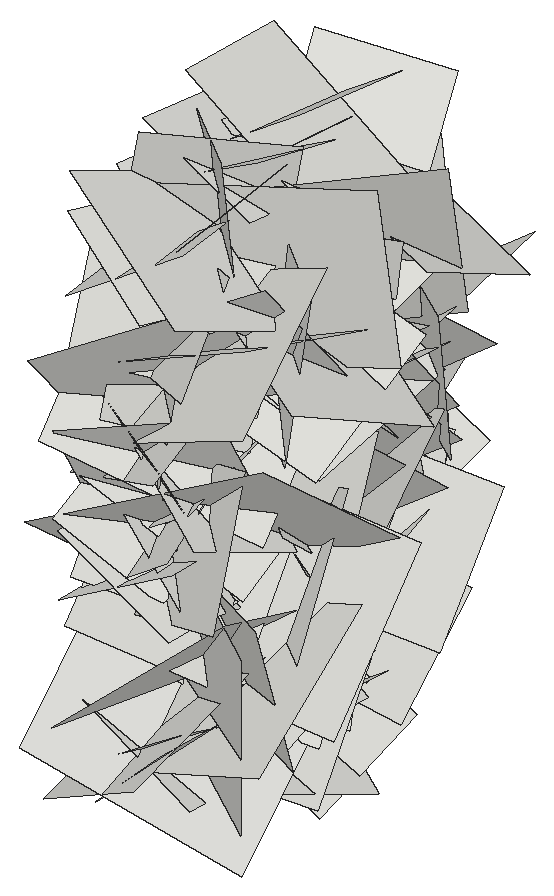
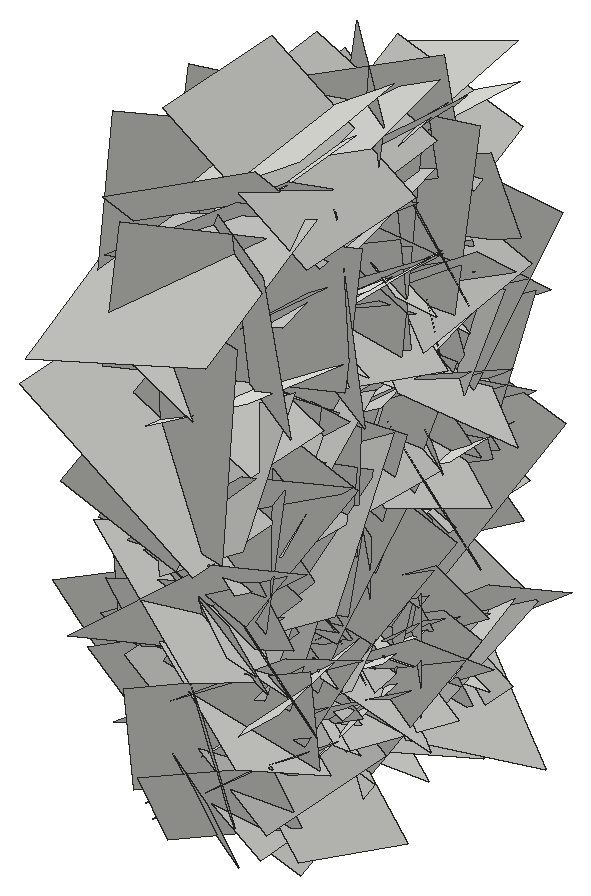
# SketchUp Ruby script. Lengths in inches.
U = 1.inch
M = Sketchup.active_model
def pt(a) = Geom::Point3d.new(a.map { |v| v * U })
def face(e, loops, mat)
  f = e.add_face(loops[0].map { |a| pt(a) })
  loops[1..].each { |l| e.add_face(l.map { |a| pt(a) }).erase! }
  f.material = f.back_material = mat if mat
  f
end
# faces: each face lists its corners as indices into pts; further lists are holes
def faces(e, pts, list, mat = nil) = list.each { |f| face(e, (f[0].is_a?(Array) ? f : [f]).map { |l| l.map { |i| pts[i] } }, mat) }
# xy, xz, yz: faces in a plane at the given z, y or x. An outline is a flat list of corners, or four numbers for a rectangle; further outlines are holes
def ring(l) = l.size == 4 ? [[l[0], l[1]], [l[2], l[1]], [l[2], l[3]], [l[0], l[3]]] : l.each_slice(2).to_a
def flat(e, list, mat, &to3) = list.each { |f| face(e, (f[0].is_a?(Array) ? f : [f]).map { |l| ring(l).map { |u, v| to3.(u, v) } }, mat) }
def xy(e, z, list, mat = nil) = flat(e, list, mat) { |x, y| [x, y, z] }
def xz(e, y, list, mat = nil) = flat(e, list, mat) { |x, z| [x, y, z] }
def yz(e, x, list, mat = nil) = flat(e, list, mat) { |y, z| [x, y, z] }
def lines(e, pts, list) = list.each { |a, b| e.add_line(pt(pts[a]), pt(pts[b])) }
# prism: a flat outline (further loops are holes) pulled along v
def prism(e, loops, v, mat = nil)
  f = face(e, loops, mat); d = Geom::Vector3d.new(v.map { |x| x * U })
  f.pushpull(f.normal.samedirection?(d) ? d.length : -d.length)
end
def box(e, o, s, mat = nil) = prism(e, [[o, [o[0] + s[0], o[1], o[2]], [o[0] + s[0], o[1] + s[1], o[2]], [o[0], o[1] + s[1], o[2]]]], [0, 0, s[2]], mat)
def at(x, y, z, deg = 0) = Geom::Transformation.translation(pt([x, y, z])) * Geom::Transformation.rotation(ORIGIN, Z_AXIS, deg.degrees)
def axes(o, x, y, z) = Geom::Transformation.new([*x, 0, *y, 0, *z, 0, *pt(o).to_a, 1])
def part(name) = M.definitions.add(name)
# library, detail: a bought-in or finely detailed component or shape, given as its bounding box
def library(name, o, s) = part(name).tap { |d| box(d.entities, o, s) }
def detail(e, o, s) = box(e.add_group.entities, o, s)
def put(e, d, t, mat = nil) = e.add_instance(d, t).tap { |i| i.material = mat if mat }
def group(e, t, mat = nil) = e.add_group.tap { |g| g.transformation = t; g.material = mat if mat }.entities
root = M.entities
c1 = part("Component\#6")
p = [[0.01,0,0],[0,3.24,4.54],[4.32,3.24,4.54],[4.33,0,0]]
faces(c1.entities,p,[[0,1,2,3]])
put(root,c1,axes([420.52,139.71,39.61],[0.08624,0.67106,-0.00672],[-0.16105,0.01183,-0.6586],[0.69289,-0.08077,-0.15225]))
put(root,c1,axes([424.49,144.65,25.96],[-0.15377,0.53431,0.65108],[-0.06081,0.65286,-0.54856],[-0.89071,-0.13681,-0.07495]))
put(root,c1,axes([420.52,144.73,33.27],[-0.16555,-0.76551,-0.15352],[0.02389,-0.16091,0.77946],[0.82725,-0.14855,-0.05323]))
put(root,c1,axes([420.52,146.45,21.25],[-0.00375,0.2874,0.54008],[0.0654,0.5375,-0.28562],[0.64519,-0.05282,0.03209]))
put(root,c1,axes([420.52,136.92,29.78],[0.03864,0.57092,0.32429],[-0.05823,0.3263,-0.56829],[0.69355,-0.00442,-0.06578]))
put(root,c1,axes([420.52,144.18,33.46],[-0.08879,-0.56105,-0.39599],[0.0694,-0.40364,0.55803],[0.72461,-0.03009,-0.10197]))
put(root,c1,axes([424.49,149.17,29.19],[-0.22051,-0.77582,-0.34275],[0.07369,-0.36732,0.78924],[-0.89602,0.16072,0.14925]))
put(root,c1,axes([420.52,141.16,33.73],[0.01034,-0.20439,-0.70125],[-0.11317,-0.69418,0.20085],[0.76594,-0.09981,0.03914]))
put(root,c1,axes([420.52,145.72,37.21],[0.0202,-0.65006,0.07365],[-0.02062,0.07308,0.65011],[0.69316,0.02112,0.01719]))
put(root,c1,axes([420.52,146.3,23.53],[-0.0913,-0.50535,0.50896],[0.05568,0.5068,0.51209],[0.75823,-0.09807,0.02368]))
put(root,c1,axes([420.52,145.7,22.51],[-0.08358,0.19729,0.79599],[-0.0899,0.79341,-0.20506],[0.86462,0.10156,0.05562]))
put(root,c1,axes([424.49,145.12,23.07],[0.0526,-0.82286,-0.58821],[-0.0059,-0.58914,0.82367],[-1.07215,-0.03713,-0.03339]))
put(root,c1,axes([424.49,137.68,27.62],[-0.00267,0.49736,0.77514],[-0.05686,0.77375,-0.49665],[-0.97459,-0.04651,0.02685]))
put(root,c1,axes([424.49,136.3,32.46],[0.17238,0.91042,0.71253],[0.07022,0.71102,-0.92361],[-1.22345,0.16908,0.04738]))
put(root,c1,axes([420.52,137.77,24.11],[-0.1419,0.78136,-0.16109],[0.04598,-0.15597,-0.79258],[0.84441,0.13979,0.01609]))
put(root,c1,axes([420.52,143.53,22.21],[-0.15224,-0.84766,-0.36991],[-0.10957,-0.35729,0.85887],[0.97421,-0.17265,0.03879]))
put(root,c1,axes([424.49,135.48,23.28],[0.21581,1.04519,0.5846],[0.09636,0.57779,-1.06467],[-1.26577,0.22219,0.01862]))
put(root,c1,axes([420.52,145.6,27.28],[0.00806,0.29423,-0.56577],[0.12293,-0.55701,-0.28812],[0.6647,0.09945,0.06014]))
put(root,c1,axes([424.49,141.63,23.18],[0.01995,1.00092,0.30572],[0.13829,0.30114,-0.99396],[-1.10071,0.05598,-0.11933]))
put(root,c1,axes([424.49,145.42,24.52],[0.2647,-0.88765,0.75819],[0.01358,0.77738,0.90589],[-1.23735,-0.18136,0.17214]))
put(root,c1,axes([420.52,144.6,22.65],[-0.17478,-0.82558,-0.09028],[0.09417,-0.10904,0.83495],[0.87528,-0.15312,-0.10786]))
put(root,c1,axes([424.49,142.67,41.25],[0.05619,0.9574,-0.08237],[-0.00834,-0.08206,-0.95886],[-1.01856,0.05349,0.00331]))
put(root,c1,axes([424.49,148.52,32.35],[-0.08011,-0.79067,-0.06214],[-0.07476,-0.05548,0.79163],[-0.83736,0.0806,-0.06473]))
put(root,c1,axes([420.52,140.84,40.56],[-0.05261,0.712,-0.12967],[0.10362,-0.12219,-0.70833],[0.7601,0.06594,0.08758]))
put(root,c1,axes([420.52,143.38,25.93],[-0.00088,-0.66729,0.07011],[0.1194,0.06898,0.65784],[0.70113,-0.01259,-0.11194]))
put(root,c1,axes([420.52,144.05,31.85],[-0.11078,0.17753,-0.74918],[0.12323,-0.74375,-0.19246],[0.80677,0.13798,-0.07348]))
put(root,c1,axes([424.49,138.53,29.67],[-0.03677,-0.4198,0.69058],[-0.10131,0.68849,0.41374],[-0.85065,-0.06385,-0.07912]))
put(root,c1,axes([424.49,150.98,27.43],[-0.11329,-0.77541,-0.3635],[0.07754,-0.37325,0.77469],[-0.90445,0.06513,0.11195]))
put(root,c1,axes([424.49,149.13,24.11],[0.03147,-0.85153,-0.39996],[0.02133,-0.3995,0.85202],[-0.997,-0.03542,0.00561]))
put(root,c1,axes([424.49,144.71,33.13],[0.16995,0.04512,1.05289],[0.00982,1.0649,-0.04705],[-1.11704,0.01623,0.15977]))
put(root,c1,axes([420.52,143.64,28.51],[0.01569,-0.00258,-0.72773],[0.02057,-0.72762,0.00297],[0.77112,0.01947,0.01473]))
put(root,c1,axes([424.49,137.85,30.84],[0.06669,0.91948,0.38333],[0.06841,0.37952,-0.92095],[-1.05374,0.08283,-0.03553]))
put(root,c1,axes([424.49,147.08,31.53],[0.0186,0.21399,-0.90436],[0.04027,-0.90393,-0.21315],[-0.98427,-0.03294,-0.02581]))
put(root,c1,axes([420.52,144.98,23.12],[0.11015,0.70988,0.06167],[-0.04855,0.06885,-0.71532],[0.75374,-0.09931,-0.05509]))
put(root,c1,axes([420.52,140.76,35.5625],[0.0095,0.80566,-0.00603],[-0.04784,-0.00552,-0.80445],[0.85268,-0.00929,-0.04507]))
put(root,c1,axes([420.52,146.7,34.04],[-0.22474,0.77203,-0.6543],[-0.03576,-0.67353,-0.78378],[1.07212,0.13937,-0.1633]))
put(root,c1,axes([424.49,141.61,27.46],[0.15544,0.8369,-0.58263],[0.03072,-0.5918,-0.84279],[-1.08048,0.10358,-0.10778]))
put(root,c1,axes([424.49,145.6875,25.3],[0.21495,-0.77208,-0.77151],[0.06755,-0.77499,0.79232],[-1.15499,-0.18901,-0.09724]))
put(root,c1,axes([424.49,147.86,21.63],[0.08807,-1.00346,0.13322],[0.11481,0.14172,0.99989],[-1.06685,-0.06759,0.1186]))
put(root,c1,axes([420.52,139.84,37.375],[0.13047,0.02824,0.77],[-0.11824,0.77221,-0.01049],[0.80815,0.10842,-0.12584]))
put(root,c1,axes([424.49,144.76,23.61],[-0.10873,-0.7568,0.02149],[0.01122,0.02025,0.76368],[-0.80245,0.10283,0.00777]))
put(root,c1,axes([420.52,149.44,28.46],[-0.01637,-0.35652,-0.61871],[0.18604,-0.60176,0.34238],[0.7337,0.14463,-0.10062]))
put(root,c1,axes([420.52,137.14,29.31],[0.00249,0.75761,-0.01469],[0.08098,-0.01485,-0.75375],[0.79913,-0.00085,0.07643]))
put(root,c1,axes([420.52,137.53,34.5],[-0.08019,0.3809,0.76753],[0.04804,0.77121,-0.37826],[0.90698,-0.00717,0.08789]))
put(root,c1,axes([424.49,139.47,36.72],[-0.15825,-0.66033,0.08813],[-0.02764,0.09604,0.67542],[-0.70562,0.14433,-0.04622]))
put(root,c1,axes([420.52,139.47,36.72],[0.15825,-0.66033,0.08813],[0.02764,0.09604,0.67542],[0.70562,0.14433,-0.04622]))
put(root,c1,axes([424.49,137.53,34.5],[0.08019,0.3809,0.76753],[-0.04804,0.77121,-0.37826],[-0.90698,-0.00717,0.08789]))
put(root,c1,axes([424.49,137.14,29.31],[-0.00249,0.75761,-0.01469],[-0.08098,-0.01485,-0.75375],[-0.79913,-0.00085,0.07643]))
put(root,c1,axes([424.49,149.44,28.46],[0.01637,-0.35652,-0.61871],[-0.18604,-0.60176,0.34238],[-0.7337,0.14463,-0.10062]))
put(root,c1,axes([420.52,144.76,23.61],[0.10873,-0.7568,0.02149],[-0.01122,0.02025,0.76368],[0.80245,0.10283,0.00777]))
put(root,c1,axes([424.49,139.84,37.375],[-0.13047,0.02824,0.77],[0.11824,0.77221,-0.01049],[-0.80815,0.10842,-0.12584]))
put(root,c1,axes([420.52,147.86,21.63],[-0.08807,-1.00346,0.13322],[-0.11481,0.14172,0.99989],[1.06685,-0.06759,0.1186]))
put(root,c1,axes([420.52,145.6875,25.3],[-0.21495,-0.77208,-0.77151],[-0.06755,-0.77499,0.79232],[1.15499,-0.18901,-0.09724]))
put(root,c1,axes([420.52,141.61,27.46],[-0.15544,0.8369,-0.58263],[-0.03072,-0.5918,-0.84279],[1.08048,0.10358,-0.10778]))
put(root,c1,axes([424.49,146.7,34.04],[0.22474,0.77203,-0.6543],[0.03576,-0.67353,-0.78378],[-1.07212,0.13937,-0.1633]))
put(root,c1,axes([424.49,140.76,35.5625],[-0.0095,0.80566,-0.00603],[0.04784,-0.00552,-0.80445],[-0.85268,-0.00929,-0.04507]))
put(root,c1,axes([424.49,144.98,23.12],[-0.11015,0.70988,0.06167],[0.04855,0.06885,-0.71532],[-0.75374,-0.09931,-0.05509]))
put(root,c1,axes([420.52,147.08,31.53],[-0.0186,0.21399,-0.90436],[-0.04027,-0.90393,-0.21315],[0.98427,-0.03294,-0.02581]))
put(root,c1,axes([420.52,137.85,30.84],[-0.06669,0.91948,0.38333],[-0.06841,0.37952,-0.92095],[1.05374,0.08283,-0.03553]))
put(root,c1,axes([424.49,143.64,28.51],[-0.01569,-0.00258,-0.72773],[-0.02057,-0.72762,0.00297],[-0.77112,0.01947,0.01473]))
put(root,c1,axes([420.52,144.71,33.13],[-0.16995,0.04512,1.05289],[-0.00982,1.0649,-0.04705],[1.11704,0.01623,0.15977]))
put(root,c1,axes([420.52,149.13,24.11],[-0.03147,-0.85153,-0.39996],[-0.02133,-0.3995,0.85202],[0.997,-0.03542,0.00561]))
put(root,c1,axes([420.52,150.98,27.43],[0.11329,-0.77541,-0.3635],[-0.07754,-0.37325,0.77469],[0.90445,0.06513,0.11195]))
put(root,c1,axes([420.52,138.53,29.67],[0.03677,-0.4198,0.69058],[0.10131,0.68849,0.41374],[0.85065,-0.06385,-0.07912]))
put(root,c1,axes([424.49,144.05,31.85],[0.11078,0.17753,-0.74918],[-0.12323,-0.74375,-0.19246],[-0.80677,0.13798,-0.07348]))
put(root,c1,axes([424.49,143.38,25.93],[0.00088,-0.66729,0.07011],[-0.1194,0.06898,0.65784],[-0.70113,-0.01259,-0.11194]))
put(root,c1,axes([424.49,140.84,40.56],[0.05261,0.712,-0.12967],[-0.10362,-0.12219,-0.70833],[-0.7601,0.06594,0.08758]))
put(root,c1,axes([420.52,148.52,32.35],[0.08011,-0.79067,-0.06214],[0.07476,-0.05548,0.79163],[0.83736,0.0806,-0.06473]))
put(root,c1,axes([420.52,142.67,41.25],[-0.05619,0.9574,-0.08237],[0.00834,-0.08206,-0.95886],[1.01856,0.05349,0.00331]))
put(root,c1,axes([424.49,144.6,22.65],[0.17478,-0.82558,-0.09028],[-0.09417,-0.10904,0.83495],[-0.87528,-0.15312,-0.10786]))
put(root,c1,axes([420.52,145.42,24.52],[-0.2647,-0.88765,0.75819],[-0.01358,0.77738,0.90589],[1.23735,-0.18136,0.17214]))
put(root,c1,axes([420.52,141.63,23.18],[-0.01995,1.00092,0.30572],[-0.13829,0.30114,-0.99396],[1.10071,0.05598,-0.11933]))
put(root,c1,axes([424.49,145.6,27.28],[-0.00806,0.29423,-0.56577],[-0.12293,-0.55701,-0.28812],[-0.6647,0.09945,0.06014]))
put(root,c1,axes([420.52,135.48,23.28],[-0.21581,1.04519,0.5846],[-0.09636,0.57779,-1.06467],[1.26577,0.22219,0.01862]))
put(root,c1,axes([424.49,143.53,22.21],[0.15224,-0.84766,-0.36991],[0.10957,-0.35729,0.85887],[-0.97421,-0.17265,0.03879]))
put(root,c1,axes([424.49,137.77,24.11],[0.1419,0.78136,-0.16109],[-0.04598,-0.15597,-0.79258],[-0.84441,0.13979,0.01609]))
put(root,c1,axes([420.52,136.3,32.46],[-0.17238,0.91042,0.71253],[-0.07022,0.71102,-0.92361],[1.22345,0.16908,0.04738]))
put(root,c1,axes([420.52,137.68,27.62],[0.00267,0.49736,0.77514],[0.05686,0.77375,-0.49665],[0.97459,-0.04651,0.02685]))
put(root,c1,axes([420.52,145.12,23.07],[-0.0526,-0.82286,-0.58821],[0.0059,-0.58914,0.82367],[1.07215,-0.03713,-0.03339]))
put(root,c1,axes([424.49,145.7,22.51],[0.08358,0.19729,0.79599],[0.0899,0.79341,-0.20506],[-0.86462,0.10156,0.05562]))
put(root,c1,axes([424.49,146.3,23.53],[0.0913,-0.50535,0.50896],[-0.05568,0.5068,0.51209],[-0.75823,-0.09807,0.02368]))
put(root,c1,axes([424.49,145.72,37.21],[-0.0202,-0.65006,0.07365],[0.02062,0.07308,0.65011],[-0.69316,0.02112,0.01719]))
put(root,c1,axes([424.49,141.16,33.73],[-0.01034,-0.20439,-0.70125],[0.11317,-0.69418,0.20085],[-0.76594,-0.09981,0.03914]))
put(root,c1,axes([420.52,149.17,29.19],[0.22051,-0.77582,-0.34275],[-0.07369,-0.36732,0.78924],[0.89602,0.16072,0.14925]))
put(root,c1,axes([424.49,144.18,33.46],[0.08879,-0.56105,-0.39599],[-0.0694,-0.40364,0.55803],[-0.72461,-0.03009,-0.10197]))
put(root,c1,axes([424.49,136.92,29.78],[-0.03864,0.57092,0.32429],[0.05823,0.3263,-0.56829],[-0.69355,-0.00442,-0.06578]))
put(root,c1,axes([424.49,146.45,21.25],[0.00375,0.2874,0.54008],[-0.0654,0.5375,-0.28562],[-0.64519,-0.05282,0.03209]))
put(root,c1,axes([424.49,144.73,33.27],[0.16555,-0.76551,-0.15352],[-0.02389,-0.16091,0.77946],[-0.82725,-0.14855,-0.05323]))
put(root,c1,axes([420.52,144.65,25.96],[0.15377,0.53431,0.65108],[0.06081,0.65286,-0.54856],[0.89071,-0.13681,-0.07495]))
put(root,c1,axes([424.49,139.71,39.61],[-0.08624,0.67106,-0.00672],[0.16105,0.01183,-0.6586],[-0.69289,-0.08077,-0.15225]))
put(root,c1,axes([420.52,143.41,32.67],[-0.00295,0.89075,-0.72818],[-0.15415,-0.72261,-0.88339],[1.20976,-0.08991,-0.11434]))
put(root,c1,axes([420.52,146.5,19.86],[0.14062,-0.87102,0.18651],[0.03259,0.19294,0.87915],[0.94365,0.12313,-0.05815]))
put(root,c1,axes([420.52,145.05,38.54],[-0.26561,0.06521,-1.32838],[-0.06869,-1.35074,-0.05408],[1.4081,-0.05359,-0.25321]))
put(root,c1,axes([420.52,142.58,23.75],[0.11698,0.88265,-0.34817],[-0.00423,-0.35009,-0.88876],[1.00576,-0.10414,0.03675]))
put(root,c1,axes([420.52,141.41,21.99],[0.04242,-1.10503,0.33762],[-0.18816,0.32793,1.09436],[1.21025,0.08972,0.15831]))
put(root,c1,axes([424.49,145.49,24.46],[0.14807,-0.32942,-0.64401],[-0.00647,-0.65643,0.33444],[-0.76675,-0.05808,-0.12719]))
put(root,c1,axes([420.52,138.75,33.42],[0.07987,0.93748,-0.3836],[-0.04246,-0.3816,-0.94046],[1.07286,-0.0849,-0.00867]))
put(root,c1,axes([424.49,142.8,24.59],[0.06246,-0.31977,0.5346],[-0.03506,0.53462,0.32343],[-0.65938,-0.05871,0.03344]))
put(root,c1,axes([424.49,142.28,27.34],[0.09885,-0.42767,0.49172],[-0.03253,0.4933,0.43487],[-0.69002,-0.08452,0.04994]))
put(root,c1,axes([420.52,139.49,21.74],[0.04906,0.46783,0.90513],[0.0041,0.90598,-0.46846],[1.08001,-0.02469,-0.03934]))
put(root,c1,axes([424.49,149.12,29.1],[0.10824,-0.19319,-0.65872],[0.02698,-0.66445,0.19881],[-0.72715,-0.05341,-0.09068]))
put(root,c1,axes([420.52,145.04,25.97],[-0.0145,-0.85349,0.83598],[-0.13626,0.83223,0.84756],[1.25903,0.08024,0.10136]))
put(root,c1,axes([424.49,141.05,35.76],[0.06877,-0.60814,0.14272],[0.00885,0.14432,0.61116],[-0.66208,-0.06124,0.02299]))
put(root,c1,axes([424.49,149.56,39.6],[0.17317,-0.50739,-0.45031],[-0.03865,-0.46908,0.51531],[-0.71806,-0.09712,-0.13634]))
put(root,c1,axes([424.49,140.39,26.94],[0.03872,-0.62994,0.14227],[0.11345,0.14643,0.62088],[-0.67508,-0.01152,0.1125]))
put(root,c1,axes([424.49,144.97,35.07],[0.07722,-0.5315,-0.34657],[0.05738,-0.34237,0.53643],[-0.67013,-0.09056,0.006]))
put(root,c1,axes([420.52,139.67,30.68],[-0.09112,-0.77438,0.96294],[-0.03313,0.96632,0.77431],[1.3094,-0.02944,0.0866]))
put(root,c1,axes([420.52,138.43,27.8],[0.10648,0.28124,1.16655],[-0.16097,1.1642,-0.2676],[1.26174,0.12479,-0.13259]))
put(root,c1,axes([420.52,140.69,35.43],[0.02714,1.22478,0.26938],[-0.1382,0.27058,-1.21783],[1.3221,0.00314,-0.13283]))
put(root,c1,axes([420.52,137.65,40.3125],[0.15365,0.92766,-0.3555],[0.07441,-0.36793,-0.93147],[1.05042,-0.10963,0.11798]))
put(root,c1,axes([424.49,136.62,23.89],[0.08859,0.63974,0.04756],[0.12242,0.03217,-0.63572],[-0.66888,0.09062,-0.11005]))
put(root,c1,axes([420.52,149.09,36.34],[-0.1737,0.35213,-1.24285],[0.08,-1.24806,-0.36356],[1.36694,0.11779,-0.13666]))
put(root,c1,axes([420.52,146.73,29.36],[-0.09029,-1.26195,0.03468],[0.03892,0.03227,1.26436],[1.33761,-0.08612,-0.03444]))
put(root,c1,axes([420.52,141.99,33.2],[0.15631,-0.03731,1.01998],[0.08418,1.02787,0.02612],[1.07863,-0.07482,-0.14985]))
put(root,c1,axes([420.52,141.2,30.22],[0.14348,-0.5033,-0.91823],[0.06175,-0.92081,0.51331],[1.10823,0.11647,0.09028]))
put(root,c1,axes([420.52,143.42,27.33],[0.08667,-0.86973,1.01008],[-0.23887,0.9884,0.86929],[1.39256,0.22367,0.08625]))
put(root,c1,axes([420.52,142.6875,32.73],[-0.11413,-1.14483,0.29443],[0.2702,0.26621,1.12831],[1.22353,-0.16558,-0.2217]))
put(root,c1,axes([420.52,143.97,23.32],[0.18437,0.48358,0.83906],[0.16998,0.82633,-0.50949],[1.01237,-0.22682,-0.06726]))
put(root,c1,axes([420.52,144,25.2],[0.04504,0.58566,0.95802],[0.11757,0.95183,-0.5868],[1.18441,-0.11675,0.02182]))
put(root,c1,axes([420.52,150.86,30.47],[0.14962,-1.13409,-0.09371],[-0.03493,-0.09847,1.14197],[1.20573,0.13788,0.04471]))
put(root,c1,axes([420.52,141.59,27.99],[-0.06396,0.08339,-1.32201],[-0.02487,-1.32324,-0.0824],[1.4039,-0.01964,-0.06169]))
put(root,c1,axes([420.52,145.76,27.48],[0.11303,-0.66031,-0.96553],[-0.02355,-0.9705,0.66125],[1.23968,0.04176,0.1006]))
put(root,c1,axes([420.52,149.48,27.53],[0.05839,-0.93868,-0.8352],[-0.07486,-0.83699,0.93604],[1.32974,-0.0059,0.08937]))
put(root,c1,axes([420.52,141.72,37.36],[0.19445,0.97106,0.50245],[-0.00165,0.50971,-0.98451],[1.15895,-0.1622,-0.0857]))
put(root,c1,axes([420.52,141.71,25.57],[-0.24627,-1.07768,0.84944],[0.21085,0.82598,1.10232],[1.43917,-0.30542,-0.01615]))
put(root,c1,axes([420.52,141.15,27.9],[0.10356,0.25866,-1.08582],[0.18317,-1.08033,-0.24181],[1.16891,0.14638,0.13409]))
put(root,c1,axes([420.52,145.83,38.68],[-0.04371,1.09164,-0.51046],[0.28885,-0.48908,-1.06793],[1.24431,0.15188,0.22998]))
put(root,c1,axes([420.52,140.25,33.3],[-0.10371,-0.10781,1.29757],[0.22808,1.282,0.12274],[1.36119,-0.22303,0.07829]))
put(root,c1,axes([420.52,139.39,34.34],[0.15089,0.92592,0.71699],[0.08883,0.71236,-0.93659],[1.23815,-0.16395,-0.02018]))
put(root,c1,axes([420.52,142.42,32.89],[0.18672,-0.42722,1.28431],[-0.1337,1.28432,0.44452],[1.42847,0.17605,-0.12627]))
put(root,c1,axes([420.52,142.63,35.02],[0.11092,-0.98462,-0.77371],[0.1183,-0.76598,0.98988],[1.32209,0.15114,-0.02366]))
put(root,c1,axes([420.52,137.42,26.21],[0.14568,0.69276,1.17725],[0.03045,1.18146,-0.69859],[1.44759,-0.09457,-0.10377]))
put(root,c1,axes([420.52,143.09,24.72],[0.05768,-1.1082,-0.74759],[0.23067,-0.73089,1.09928],[1.3981,0.16631,-0.15052]))
put(root,c1,axes([420.52,141,38.04],[0.14868,1.2474,-0.57055],[0.09146,-0.58042,-1.24775],[1.45112,-0.09122,0.1371]))
